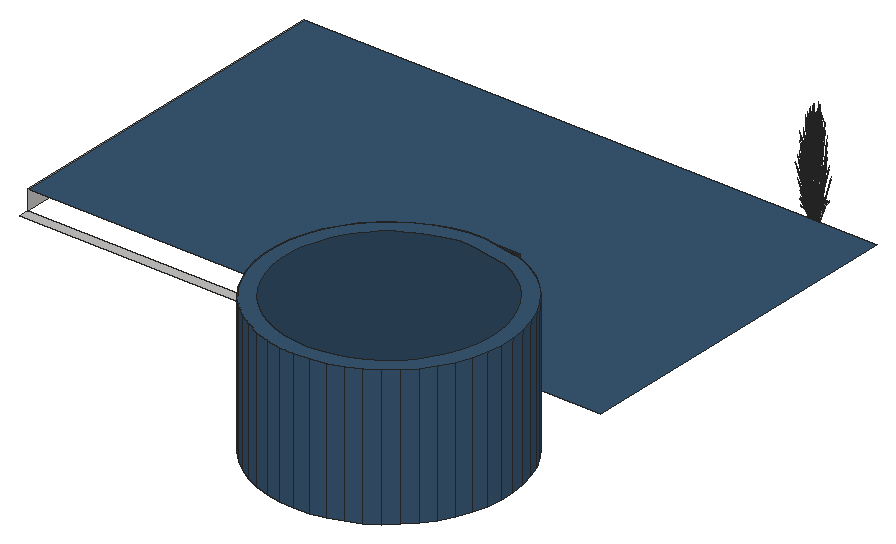
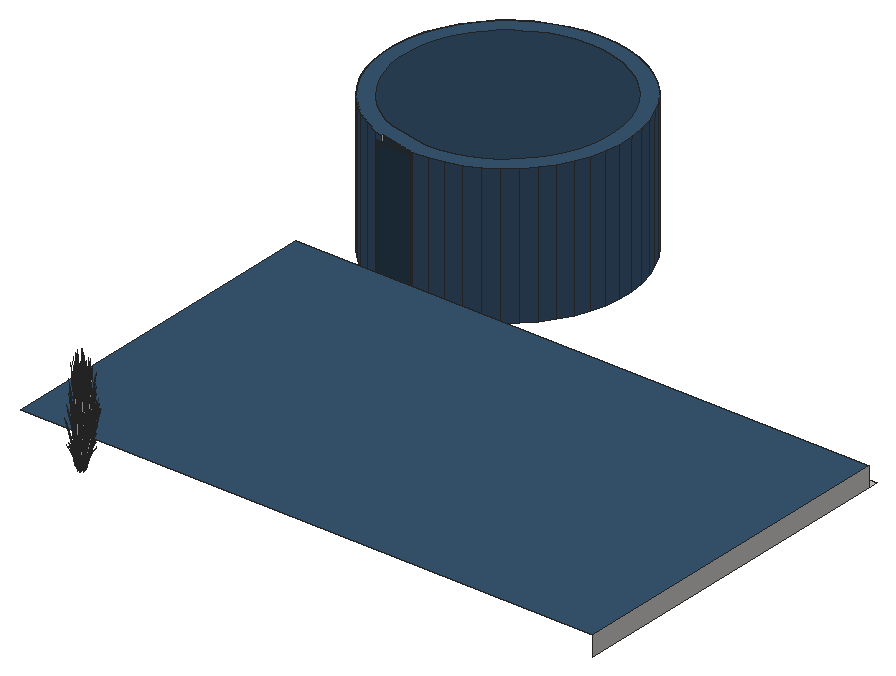
# SketchUp Ruby script. Lengths in inches.
U = 1.inch
M = Sketchup.active_model
def pt(a) = Geom::Point3d.new(a.map { |v| v * U })
def face(e, loops, mat)
  f = e.add_face(loops[0].map { |a| pt(a) })
  loops[1..].each { |l| e.add_face(l.map { |a| pt(a) }).erase! }
  f.material = f.back_material = mat if mat
  f
end
# faces: each face lists its corners as indices into pts; further lists are holes
def faces(e, pts, list, mat = nil) = list.each { |f| face(e, (f[0].is_a?(Array) ? f : [f]).map { |l| l.map { |i| pts[i] } }, mat) }
# xy, xz, yz: faces in a plane at the given z, y or x. An outline is a flat list of corners, or four numbers for a rectangle; further outlines are holes
def ring(l) = l.size == 4 ? [[l[0], l[1]], [l[2], l[1]], [l[2], l[3]], [l[0], l[3]]] : l.each_slice(2).to_a
def flat(e, list, mat, &to3) = list.each { |f| face(e, (f[0].is_a?(Array) ? f : [f]).map { |l| ring(l).map { |u, v| to3.(u, v) } }, mat) }
def xy(e, z, list, mat = nil) = flat(e, list, mat) { |x, y| [x, y, z] }
def xz(e, y, list, mat = nil) = flat(e, list, mat) { |x, z| [x, y, z] }
def yz(e, x, list, mat = nil) = flat(e, list, mat) { |y, z| [x, y, z] }
def lines(e, pts, list) = list.each { |a, b| e.add_line(pt(pts[a]), pt(pts[b])) }
# prism: a flat outline (further loops are holes) pulled along v
def prism(e, loops, v, mat = nil)
  f = face(e, loops, mat); d = Geom::Vector3d.new(v.map { |x| x * U })
  f.pushpull(f.normal.samedirection?(d) ? d.length : -d.length)
end
def box(e, o, s, mat = nil) = prism(e, [[o, [o[0] + s[0], o[1], o[2]], [o[0] + s[0], o[1] + s[1], o[2]], [o[0], o[1] + s[1], o[2]]]], [0, 0, s[2]], mat)
def at(x, y, z, deg = 0) = Geom::Transformation.translation(pt([x, y, z])) * Geom::Transformation.rotation(ORIGIN, Z_AXIS, deg.degrees)
def axes(o, x, y, z) = Geom::Transformation.new([*x, 0, *y, 0, *z, 0, *pt(o).to_a, 1])
def part(name) = M.definitions.add(name)
# library, detail: a bought-in or finely detailed component or shape, given as its bounding box
def library(name, o, s) = part(name).tap { |d| box(d.entities, o, s) }
def detail(e, o, s) = box(e.add_group.entities, o, s)
def put(e, d, t, mat = nil) = e.add_instance(d, t).tap { |i| i.material = mat if mat }
def group(e, t, mat = nil) = e.add_group.tap { |g| g.transformation = t; g.material = mat if mat }.entities
root = M.entities
M.materials.add("Carpet_01_1K").color = [196, 195, 193]
M.materials.add("Carpet_04_1K").color = [56, 85, 112]
M.materials.add("Carpet_04_1K1").color = [43, 65, 85]
M.materials.add("LightPink_Translucent").color = [144, 107, 117]
M.materials["LightPink_Translucent"].alpha = 0.75
c1 = part("blade")
p = [[2.15,0.21,22],[0,0.17,0],[0.09,0.45,0],[2.18,0.31,22],[2.29,0.31,22],[0.38,0.45,0],
  [2.48,0.24,33],[2.49,0.24,33],[2.48,0.22,33]]
faces(c1.entities,p,[[0,1,2,3],[4,5,2,3],[6,3,4,7],[8,0,3,6]])
c2 = part("seeds")
p = [[0.3,-0.1,1.38],[-0.01,-0.03,1.59],[-0.01,-0.03,0.03],[0.14,-0.07,-0.07],[0.29,-0.03,3],[0.15,0.01,3.11]]
faces(c2.entities,p,[[0,1,2,3],[1,0,4,5]],"LightPink_Translucent")
c3 = part("blade with seeds")
put(c3.entities,c1,at(0,0,0))
put(c3.entities,c2,axes([2.4,0.25,30.99],[1.5799,-0.05474,1.17369],[-0.12525,1.92788,0.29478],[-0.07173,-0.02425,1.56792]))
xy(root,1398,[[330.57,149.5,330.57,150.21,326.6875,151.48,317.8,153.17,311.55,153.5625,309.76,153.55],[330.57,150.21,330.57,153.74,311.55,153.5625,317.8,153.17,326.6875,151.48],[309.76,153.55,311.55,153.5625,308.78,153.74],[311.55,153.5625,330.57,153.74,308.78,153.74]])
xy(root,1398,[[186.57,149.5,308.78,153.74,330.57,153.74,330.57,155.5,30.57,155.5,30.57,149.51,186.57,149.51]],"Carpet_01_1K")
xy(root,1410,[[30.57,155.5,378.57,364.54]],"Carpet_04_1K")
xy(root,1482,[[[308.78,9.74,317.8,10.31,326.6875,12,335.29,14.79,343.47,18.64,351.1,23.49,358.07,29.25,364.26,35.84,369.57,43.16,373.93,51.08,377.26,59.49,379.51,68.25,380.64,77.22,380.64,86.26,379.51,95.23,377.26,103.99,373.93,112.39,369.57,120.32,364.26,127.63,358.07,134.22,351.1,139.99,343.47,144.83,335.29,148.68,330.57,150.21,330.57,149.5,308.78,153.74,299.76,153.17,290.875,151.48,282.28,148.68,274.09,144.83,266.46,139.99,259.49,134.22,253.3,127.63,247.99,120.32,243.63,112.39,240.3,103.99,238.06,95.23,236.92,86.26,236.92,77.22,238.06,68.25,240.3,59.49,243.63,51.08,247.99,43.16,253.3,35.84,259.49,29.25,266.46,23.49,274.09,18.64,282.28,14.79,290.875,12,299.76,10.31],[308.78,18.76,300.89,19.25,293.12,20.73,285.6,23.18,278.4375,26.55,271.76,30.78,265.67,35.83,260.25,41.59,255.6,47.99,251.79,54.92,248.88,62.28,246.91,69.9375,245.92,77.78,245.92,85.69,246.91,93.54,248.88,101.2,251.79,108.55,255.6,115.49,260.25,121.88,265.67,127.65,271.76,132.69,278.4375,136.93,285.6,140.3,293.12,142.74,300.89,144.22,308.19,144.68,332.82,139.9,339.12,136.93,345.8,132.69,351.89,127.65,357.31,121.88,361.96,115.49,365.77,108.55,368.68,101.2,370.65,93.54,371.64,85.69,371.64,77.78,370.65,69.9375,368.68,62.28,365.77,54.92,361.96,47.99,357.31,41.59,351.89,35.83,345.8,30.78,339.12,26.55,331.97,23.18,324.44,20.73,316.67,19.25]]],"Carpet_04_1K")
xy(root,1482,[[308.78,18.76,316.67,19.25,324.44,20.73,331.97,23.18,339.12,26.55,345.8,30.78,351.89,35.83,357.31,41.59,361.96,47.99,365.77,54.92,368.68,62.28,370.65,69.9375,371.64,77.78,371.64,85.69,370.65,93.54,368.68,101.2,365.77,108.55,361.96,115.49,357.31,121.88,351.89,127.65,345.8,132.69,339.12,136.93,332.82,139.9,308.19,144.68,300.89,144.22,293.12,142.74,285.6,140.3,278.4375,136.93,271.76,132.69,265.67,127.65,260.25,121.88,255.6,115.49,251.79,108.55,248.88,101.2,246.91,93.54,245.92,85.69,245.92,77.78,246.91,69.9375,248.88,62.28,251.79,54.92,255.6,47.99,260.25,41.59,265.67,35.83,271.76,30.78,278.4375,26.55,285.6,23.18,293.12,20.73,300.89,19.25]],"Carpet_04_1K1")
yz(root,30.57,[[155.5,1398,364.54,1410]],"Carpet_01_1K")
yz(root,236.92,[[77.22,1398,86.26,1482]],"Carpet_04_1K")
yz(root,330.57,[[149.5,1398,150.21,1482]])
yz(root,380.64,[[77.22,1398,86.26,1482]],"Carpet_04_1K")
p = [[299.76,10.31,1482],[299.76,10.31,1398],[308.78,9.74,1398],[308.78,9.74,1482],[317.8,10.31,1398],[317.8,10.31,1482],
  [290.875,12,1482],[290.875,12,1398],[326.6875,12,1398],[326.6875,12,1482],[282.28,14.79,1482],[282.28,14.79,1398],
  [335.29,14.79,1398],[335.29,14.79,1482],[274.09,18.64,1482],[274.09,18.64,1398],[343.47,18.64,1398],[343.47,18.64,1482],
  [266.46,23.49,1482],[266.46,23.49,1398],[351.1,23.49,1398],[351.1,23.49,1482],[259.49,29.25,1482],[259.49,29.25,1398],
  [358.07,29.25,1398],[358.07,29.25,1482],[253.3,35.84,1482],[253.3,35.84,1398],[364.26,35.84,1398],[364.26,35.84,1482],
  [247.99,43.16,1482],[247.99,43.16,1398],[369.57,43.16,1398],[369.57,43.16,1482],[243.63,51.08,1482],[243.63,51.08,1398],
  [373.93,51.08,1398],[373.93,51.08,1482],[240.3,59.49,1482],[240.3,59.49,1398],[377.26,59.49,1398],[377.26,59.49,1482],
  [238.06,68.25,1482],[238.06,68.25,1398],[379.51,68.25,1398],[379.51,68.25,1482],[236.92,77.22,1482],[236.92,77.22,1398],
  [380.64,77.22,1398],[380.64,77.22,1482],[238.06,95.23,1482],[238.06,95.23,1398],[236.92,86.26,1398],[236.92,86.26,1482],
  [380.64,86.26,1482],[380.64,86.26,1398],[379.51,95.23,1398],[379.51,95.23,1482],[240.3,103.99,1482],[240.3,103.99,1398],
  [377.26,103.99,1398],[377.26,103.99,1482],[243.63,112.39,1482],[243.63,112.39,1398],[373.93,112.39,1398],[373.93,112.39,1482],
  [247.99,120.32,1482],[247.99,120.32,1398],[369.57,120.32,1398],[369.57,120.32,1482],[253.3,127.63,1482],[253.3,127.63,1398],
  [364.26,127.63,1398],[364.26,127.63,1482],[259.49,134.22,1482],[259.49,134.22,1398],[358.07,134.22,1398],[358.07,134.22,1482],
  [266.46,139.99,1482],[266.46,139.99,1398],[351.1,139.99,1398],[351.1,139.99,1482],[274.09,144.83,1482],[274.09,144.83,1398],
  [343.47,144.83,1398],[343.47,144.83,1482],[282.28,148.68,1482],[282.28,148.68,1398],[335.29,148.68,1398],[335.29,148.68,1482],
  [290.875,151.48,1482],[290.875,151.48,1398],[330.57,150.21,1398],[330.57,150.21,1482],[330.57,149.5,1398],[309.76,153.55,1398],
  [309.76,153.55,1399],[329.59,149.69,1399],[329.59,149.69,1481],[309.76,153.55,1481],[308.78,153.74,1398],[308.78,153.74,1482],
  [330.57,149.5,1482],[299.76,153.17,1482],[299.76,153.17,1398],[330.57,153.74,1398],[311.55,153.5625,1398],[330.57,153.74,1481],
  [310.76,153.56,1480],[310.76,153.56,1399],[311.55,153.5625,1399],[329.58,153.73,1399],[329.58,153.73,1480]]
faces(root,p,[[0,1,2,3],[3,2,4,5],[6,7,1,0],[5,4,8,9],[10,11,7,6],[9,8,12,13],[14,15,11,10],[13,12,16,17],
  [18,19,15,14],[17,16,20,21],[22,23,19,18],[21,20,24,25],[26,27,23,22],[25,24,28,29],[30,31,27,26],[29,28,32,33],
  [34,35,31,30],[33,32,36,37],[38,39,35,34],[37,36,40,41],[42,43,39,38],[41,40,44,45],[46,47,43,42],[45,44,48,49],
  [50,51,52,53],[54,55,56,57],[58,59,51,50],[57,56,60,61],[62,63,59,58],[61,60,64,65],[66,67,63,62],[65,64,68,69],
  [70,71,67,66],[69,68,72,73],[74,75,71,70],[73,72,76,77],[78,79,75,74],[77,76,80,81],[82,83,79,78],[81,80,84,85],
  [86,87,83,82],[85,84,88,89],[90,91,87,86],[89,88,92,93],[103,104,91,90],[101,100,104,103]],"Carpet_04_1K")
faces(root,p,[[94,95,96,97,98,99,96,95,100,101,102],[[105,106,95,96,99,107],[108,109,110,111,112]],[96,99,98,97],[109,108,112,111,110]],"Carpet_04_1K1")
put(root,c3,axes([330.27,376.06,1401.875],[0.08068,0.14973,1.71376],[-0.3728,0.12606,0.13857],[-0.08426,-0.23506,0.73262]))
put(root,c3,axes([330.89,375.07,1402.72],[-0.05398,-0.06539,1.74944],[-0.36026,0.04145,-0.27667],[-0.0575,-0.15639,0.14031]))
put(root,c3,axes([331.72,375.84,1400.59],[-0.10032,0.0944,1.43002],[-0.30046,-0.16522,-0.30754],[0.05569,-0.20547,0.61141]))
put(root,c3,axes([331.27,376.17,1402.98],[-0.16845,-0.3792,-0.71045],[0.34676,-0.21133,0.08574],[-0.03939,-0.18322,1.00501]))
put(root,c3,axes([330.17,375.66,1400.59],[-0.02137,0.15256,1.43002],[-0.31245,0.12771,-0.30754],[-0.07303,-0.19719,0.61141]))
put(root,c3,axes([330.98,375.33,1399.49],[-0.0592,0.0168,1.76342],[-0.32738,-0.18913,-0.26939],[0.00549,-0.15776,0.30037]))
put(root,c3,axes([331.97,376.54,1402.98],[0.00918,-0.43138,-0.71045],[0.38672,0.02897,0.08574],[0.04081,-0.18275,1.00501]))
put(root,c3,axes([332.51,375.87,1402.72],[-0.00341,-0.09282,1.74944],[-0.28775,-0.26825,-0.27667],[0.04449,-0.16261,0.14031]))
put(root,c3,axes([331.3,375.85,1402.53],[0.1064,-0.35863,-0.35414],[0.31043,0.1046,0.4572],[-0.02846,-0.14439,0.87481]))
put(root,c3,axes([331.53,376.32,1401.875],[-0.06572,0.16029,1.71376],[-0.27569,-0.33172,0.13857],[0.12437,-0.20675,0.73262]))
put(root,c3,axes([332.43,375.53,1402.71],[-0.03584,0.03562,1.77383],[-0.35118,-0.12018,-0.16761],[-0.01271,-0.15545,0.31391]))
put(root,c3,axes([331.14,376.09,1402.68],[-0.34695,-0.11691,-0.51099],[0.11892,-0.40083,-0.3958],[-0.03181,-0.16138,0.97773]))
put(root,c3,axes([331.35,375.09,1400.77],[0.04528,0.27194,1.1486],[-0.25117,-0.15062,0.84392],[0.02703,-0.13924,0.25299]))
put(root,c3,axes([331.89,376.4,1402.68],[-0.25266,-0.31335,-0.51099],[0.2669,-0.27442,-0.3958],[0.03844,-0.15921,0.97773]))
put(root,c3,axes([330.52,374.85,1402.71],[-0.00658,0.0559,1.77383],[-0.32474,0.20287,-0.16761],[-0.09556,-0.1037,0.31391]))
put(root,c3,axes([330.45,375.84,1403.09],[0.39316,-0.11987,0.53763],[0.06823,0.47021,0.4433],[-0.09247,-0.13858,1.11249]))
put(root,c3,axes([331.34,375.93,1402.73],[0.34777,0.12192,0.48003],[-0.11892,0.40083,0.3958],[-0.0209,-0.15763,0.9933]))
put(root,c3,axes([331.4375,376.08,1403.03],[-0.34538,0.21713,-0.1216],[-0.16972,-0.38536,-0.67495],[-0.04557,-0.16239,1.02557]))
put(root,c3,axes([332.15,376.5625,1403.03],[-0.3879,-0.02311,-0.1216],[0.0106,-0.43749,-0.67495],[0.02694,-0.1685,1.02557]))
put(root,c3,axes([332.13,376.28,1402.53],[0.23881,-0.24554,-0.35414],[0.22606,0.28036,0.4572],[0.0344,-0.14245,0.87481]))
put(root,c3,axes([330.0625,375.42,1400.77],[0.18411,0.16231,1.1486],[-0.26813,0.09757,0.84392],[-0.05737,-0.12474,0.25299]))
put(root,c3,axes([331.43,375.9,1402.73],[0.26007,-0.1585,0.0643],[0.12729,0.28902,0.50621],[-0.02512,-0.1274,0.77189]))
put(root,c3,axes([330.51,376.28,1402.98],[-0.30095,-0.22541,-0.71045],[0.21388,-0.395,0.08574],[-0.10904,-0.13459,1.00501]))
put(root,c3,axes([330.4,375.98,1402.53],[-0.05451,-0.37564,-0.35414],[0.31161,-0.09919,0.4572],[-0.0837,-0.10765,0.87481]))
put(root,c3,axes([330.54,375.95,1402.73],[0.16041,-0.29625,0.0643],[0.22843,0.17248,0.50621],[-0.07385,-0.09498,0.77189]))
put(root,c3,axes([329.92,375.91,1399.49],[-0.03419,0.06144,1.76342],[-0.3455,0.13246,-0.26939],[-0.08346,-0.12049,0.30037]))
put(root,c3,axes([330.49,377.59,1400.1],[-0.14494,-0.47823,-0.69835],[0.41752,-0.17223,-0.18329],[-0.01602,-0.16194,1.54149]))
put(root,c3,axes([329.73,376.53,1401.875],[0.1311,0.08035,1.71376],[-0.27131,0.33708,0.13857],[-0.16909,-0.15206,0.73262]))
put(root,c3,axes([332.43,376.13,1399.49],[-0.05283,-0.03674,1.76342],[-0.13569,-0.41045,-0.26939],[0.09154,-0.11138,0.30037]))
put(root,c3,axes([331.33,376.23,1403.05],[-0.1064,0.35863,0.35414],[-0.31043,-0.1046,-0.4572],[-0.02846,-0.14439,0.87481]))
put(root,c3,axes([330.37,376.29,1402.68],[-0.34827,0.11086,-0.51099],[-0.06092,-0.41983,-0.3958],[-0.09354,-0.12031,0.97773]))
put(root,c3,axes([332.125,376.38,1402.73],[0.25132,0.3182,0.48003],[-0.2669,0.27442,0.3958],[0.04636,-0.14929,0.9933]))
put(root,c3,axes([330.61,375.91,1403.43],[-0.23555,0.44708,-0.13619],[-0.34112,-0.25757,-0.75594],[-0.11858,-0.12631,1.14864]))
put(root,c3,axes([332.22,376.41,1402.73],[0.29004,0.02173,0.0643],[-0.00795,0.32812,0.50621],[0.03035,-0.12569,0.77189]))
put(root,c3,axes([332,376.63,1403.05],[-0.23881,0.24554,0.35414],[-0.22606,-0.28036,-0.4572],[0.0344,-0.14245,0.87481]))
put(root,c3,axes([332.42,377.29,1402.98],[0.18436,-0.36797,-0.71045],[0.32306,0.26151,0.08574],[0.11008,-0.13332,1.00501]))
put(root,c3,axes([330.43,376.22,1400.375],[-0.22066,-0.46731,0],[0.36918,-0.26061,-0.51607],[0.08408,-0.05936,1.63711]))
put(root,c3,axes([332.41,377.12,1402.68],[-0.09067,-0.42583,-0.51099],[0.34336,-0.07449,-0.3958],[0.0984,-0.11438,0.97773]))
put(root,c3,axes([330.92,375.66,1400.13],[-0.2439,0.26754,-0.03893],[-0.22348,-0.29302,-0.17649],[-0.01573,-0.08303,0.58215]))
put(root,c3,axes([329.71,375.79,1402.72],[-0.07594,-0.00329,1.74944],[-0.24177,0.32918,-0.27667],[-0.129,-0.06726,0.14031]))
put(root,c3,axes([332.58,377.42,1403.03],[-0.32648,-0.25715,-0.1216],[0.18809,-0.3724,-0.67495],[0.09224,-0.12945,1.02557]))
put(root,c3,axes([331.23,378.83,1401.33],[0.305,0.18805,1.51261],[-0.29879,0.40513,0.59816],[-0.13384,-0.24012,1.26806]))
put(root,c3,axes([330.59,376.29,1403.05],[0.05451,0.37564,0.35414],[-0.31161,0.09919,-0.4572],[-0.0837,-0.10765,0.87481]))
put(root,c3,axes([329.63,377.53,1400.02],[0,-0.46636,-0.49651],[0.39487,0,0],[0,-0.10622,1.57504]))
put(root,c3,axes([330.73,376.15,1400.02],[0.33032,-0.23318,-0.49651],[0.19744,0.41812,0],[0.07523,-0.05311,1.57504]))
put(root,c3,axes([332.69,376.95,1400.59],[-0.12609,-0.01381,1.43002],[-0.12917,-0.37055,-0.30754],[0.1549,-0.10482,0.61141]))
put(root,c3,axes([329.65,376.53,1403.09],[0.29147,-0.34417,0.53763],[0.25138,0.3655,0.4433],[-0.13675,-0.06349,1.11249]))
put(root,c3,axes([333.38,377.3125,1402.71],[-0.0461,-0.00354,1.77383],[-0.19143,-0.37951,-0.16761],[0.07688,-0.12478,0.31391]))
put(root,c3,axes([331.12,377.1,1400.06],[0.23773,-0.35053,-0.62353],[0.29532,0.31785,-0.16365],[0.09526,-0.08744,1.37633]))
put(root,c3,axes([332.84,376.27,1400.77],[-0.11756,0.2374,1.1486],[-0.10105,-0.31895,0.84392],[0.09709,-0.07992,0.25299]))
put(root,c3,axes([332.67,377.16,1402.53],[0.30722,-0.06665,-0.35414],[0.08112,0.381,0.4572],[0.08804,-0.10234,0.87481]))
put(root,c3,axes([329.78,376.53,1402.73],[0.01777,-0.35463,0.0643],[0.26836,0.00972,0.50621],[-0.1028,-0.03711,0.77189]))
put(root,c3,axes([330.71,377.72,1400.21],[0.17124,-0.42022,-0.44739],[0.35581,0.20224,0.21531],[0,-0.09687,1.43643]))
put(root,c3,axes([329.68,376.64,1402.53],[-0.20082,-0.29199,-0.35414],[0.2293,-0.2764,0.4572],[-0.1165,-0.04206,0.87481]))
put(root,c3,axes([330.86,377.51,1400.67],[-0.04113,-0.53214,-0.29095],[0.42835,-0.03218,-0.50002],[0.07543,-0.07088,1.59708]))
put(root,c3,axes([329.8,377.54,1400.03],[0.24637,-0.29097,-0.30978],[0.24637,0.29097,0.30978],[0,-0.09372,1.38974]))
put(root,c3,axes([329.7,376.14,1400.13],[-0.10181,0.3808,-0.03893],[-0.31336,-0.11714,-0.17649],[-0.04758,-0.06228,0.58215]))
put(root,c3,axes([332.42,377.39,1403.05],[-0.30722,0.06665,0.35414],[-0.08112,-0.381,-0.4572],[0.08804,-0.10234,0.87481]))
put(root,c3,axes([330.67,378.07,1400.67],[-0.39748,-0.22252,-0.29095],[0.19139,-0.46966,-0.50002],[-0.01249,-0.11531,1.59708]))
put(root,c3,axes([329.53,377.88,1400.375],[-0.44133,0,0],[0,-0.52122,-0.51607],[0,-0.11871,1.63711]))
put(root,c3,axes([329.61,376.95,1400.59],[0.06891,0.12984,1.43002],[-0.15879,0.35293,-0.30754],[-0.16304,-0.08436,0.61141]))
put(root,c3,axes([330.81,376.33,1400.03],[0.32928,0.11539,-0.30978],[-0.08291,0.40636,0.30978],[0.06638,-0.04686,1.38974]))
put(root,c3,axes([329.89,376.84,1402.98],[-0.35281,-0.01123,-0.71045],[0.0237,-0.47284,0.08574],[-0.14947,-0.0499,1.00501]))
put(root,c3,axes([332.7,377.33,1402.73],[0.2423,0.19613,0.0643],[-0.14107,0.2793,0.50621],[0.07768,-0.0903,0.77189]))
put(root,c3,axes([332.63,377.25,1402.73],[0.08753,0.42921,0.48003],[-0.34336,0.07449,0.3958],[0.1012,-0.10094,0.9933]))
put(root,c3,axes([333.55,377.77,1402.72],[0.04898,-0.07104,1.74944],[-0.06269,-0.43574,-0.27667],[0.12289,-0.08262,0.14031]))
put(root,c3,axes([329.875,377.74,1400.33],[-0.32829,0.39208,0.30756],[-0.32849,-0.38796,-0.36492],[-0.01146,-0.11134,1.64885]))
put(root,c3,axes([329.42,376.07,1402.71],[0.02617,0.04654,1.77383],[-0.12614,0.41836,-0.16761],[-0.12775,0.00303,0.31391]))
put(root,c3,axes([330.92,377.93,1400.43],[0.39767,0.22603,0.24065],[-0.19139,0.46966,0.50002],[0,-0.10827,1.60543]))
put(root,c3,axes([330.77,378.5625,1400.4375],[0.09355,-0.55261,-0.23429],[0.44354,0.09633,0.51271],[-0.0775,-0.07631,1.5644]))
put(root,c3,axes([329.78,376.93,1402.68],[-0.25628,0.30892,-0.51099],[-0.22444,-0.32634,-0.3958],[-0.13021,-0.047,0.97773]))
put(root,c3,axes([329.97,376.79,1403.05],[0.20082,0.29199,0.35414],[-0.2293,0.2764,-0.4572],[-0.1165,-0.04206,0.87481]))
put(root,c3,axes([329.2,377.34,1400.77],[0.22533,-0.03337,1.1486],[-0.14293,0.29403,0.84392],[-0.11135,-0.04411,0.25299]))
put(root,c3,axes([330.79,377.61,1400.72],[-0.38326,0.02879,0.44739],[-0.03466,-0.47788,-0.21531],[0.06861,-0.04843,1.43643]))
put(root,c3,axes([329.91,376.61,1403.03],[-0.0189,0.47427,-0.1216],[-0.35781,-0.01296,-0.67495],[-0.13781,-0.03295,1.02557]))
put(root,c3,axes([329.8,377.96,1400.48],[0,0.46636,0.49651],[-0.39487,0,0],[0,-0.10622,1.57504]))
put(root,c3,axes([332.59,378.43,1403.03],[-0.17758,-0.42229,-0.1216],[0.31518,-0.20752,-0.67495],[0.13282,-0.05572,1.02557]))
put(root,c3,axes([332.57,378.06,1402.68],[0.09562,-0.42421,-0.51099],[0.32782,0.1454,-0.3958],[0.13199,-0.0389,0.97773]))
put(root,c3,axes([332.06,376.34,1400.375],[0.22066,-0.46731,0],[0.36918,0.26061,-0.51607],[0.08408,0.05936,1.63711]))
put(root,c3,axes([329.46,377.26,1401.875],[0.14639,-0.01056,1.71376],[-0.09712,0.45778,0.13857],[-0.20862,-0.02831,0.73262]))
put(root,c3,axes([330.73,378.34,1400.21],[-0.21202,-0.39143,-0.44739],[0.32115,-0.27564,0.21531],[-0.06861,-0.04843,1.43643]))
put(root,c3,axes([330.78,377.78,1400.36],[0.15345,0.52148,0.45755],[-0.43845,0.18134,0.17955],[0.00536,-0.09582,1.58856]))
put(root,c3,axes([332.92,378.18,1399.98],[-0.22732,0.05597,1.41583],[-0.03618,-0.44548,0.08104],[0.15921,-0.06743,0.80566]))
put(root,c3,axes([333.34,377.79,1400.26],[-0.21881,-0.29821,-0.06488],[0.23965,-0.27324,-0.29416],[0.0679,-0.01924,0.97024]))
put(root,c3,axes([330.7,378.2,1400.72],[-0.17124,0.42022,0.44739],[-0.35581,-0.20224,-0.21531],[0,-0.09687,1.43643]))
put(root,c3,axes([331.33,377.83,1400.21],[0,-0.53961,0],[0.44133,0,0],[0,0,1.79456]))
put(root,c3,axes([331.87,376.58,1400.48],[-0.33032,-0.23318,0.49651],[0.19744,-0.41812,0],[0.07523,0.05311,1.57504]))
put(root,c3,axes([332.51,378.22,1402.98],[0.31014,-0.20596,-0.71045],[0.17284,0.42397,0.08574],[0.14985,-0.04816,1.00501]))
put(root,c3,axes([330.54,378.49,1400.06],[-0.36714,-0.07646,-0.62353],[0.07747,-0.47163,-0.16365],[-0.10956,-0.05715,1.37633]))
put(root,c3,axes([331.12,377.49,1400.36],[-0.29264,0.42323,0.45755],[-0.34767,-0.3736,0.17955],[0.07055,-0.04224,1.58856]))
put(root,c3,axes([331.44,378.25,1400.3],[-0.32829,-0.4014,-0.06131],[0.32849,-0.40164,0],[-0.01146,-0.01402,1.75571]))
put(root,c3,axes([330.61,376.79,1400.47],[-0.10196,0.46348,0.17642],[-0.3731,-0.13116,0.35086],[0.06445,-0.00226,1.60407]))
put(root,c3,axes([332.47,378.3,1403.05],[-0.29332,-0.1301,0.35414],[0.08555,-0.37955,-0.4572],[0.11809,-0.0348,0.87481]))
put(root,c3,axes([329.4,377.61,1402.73],[0.09971,-0.42522,0.48003],[0.32782,0.1454,0.3958],[-0.12892,0.02555,0.9933]))
put(root,c3,axes([330.46,377.17,1399.59],[-0.3474,0.18671,1.28929],[-0.11057,-0.53572,0.50096],[0.21332,0.00891,1.46642]))
put(root,c3,axes([331.39,377.31,1400.62],[0.06809,-0.4162,0.1448],[0.33266,0.07225,-0.41347],[0.06054,0.04274,1.26744]))
put(root,c3,axes([329.37,377.49,1402.73],[-0.12963,-0.31798,0.0643],[0.23638,-0.15564,0.50621],[-0.1042,0.03071,0.77189]))
put(root,c3,axes([330.82,378.3,1400.36],[0.44609,0.09826,0.45755],[-0.09078,0.55493,0.17955],[-0.06519,-0.05359,1.58856]))
put(root,c3,axes([333.17,377.89,1399.49],[-0.01845,-0.0708,1.76342],[0.12793,-0.41416,-0.26939],[0.12905,-0.00596,0.30037]))
put(root,c3,axes([329.36,377.82,1399.49],[0.00895,0.0735,1.76342],[-0.18044,0.38382,-0.26939],[-0.12817,-0.01935,0.30037]))
put(root,c3,axes([331.25,377.42,1400.72],[-0.21202,-0.39143,0.44739],[0.32115,-0.27564,-0.21531],[0.06861,0.04843,1.43643]))
put(root,c3,axes([330.15,379.21,1400.03],[-0.08291,-0.40636,-0.30978],[0.32928,-0.11539,0.30978],[-0.06638,-0.04686,1.38974]))
put(root,c3,axes([330.58,379.18,1400.47],[0.37926,-0.12378,0.17642],[0.09365,0.46065,0.35086],[-0.03382,-0.06712,1.60407]))
put(root,c3,axes([331.36,377.44,1400.67],[0.35635,-0.30962,-0.29095],[0.23697,0.43749,-0.50002],[0.08792,0.04443,1.59708]))
put(root,c3,axes([332.78,378.26,1402.53],[0.29332,0.1301,-0.35414],[-0.08555,0.37955,0.4572],[0.11809,-0.0348,0.87481]))
put(root,c3,axes([330.0625,379.38,1400.02],[-0.33032,-0.23318,-0.49651],[0.19744,-0.41812,0],[-0.07523,-0.05311,1.57504]))
put(root,c3,axes([332.26,376.62,1400.02],[0.33032,0.23318,-0.49651],[-0.19744,0.41812,0],[0.07523,0.05311,1.57504]))
put(root,c3,axes([329.33,377.65,1402.53],[-0.29332,-0.1301,-0.35414],[0.08555,-0.37955,0.4572],[-0.11809,0.0348,0.87481]))
put(root,c3,axes([331.63,377.95,1400.21],[0.39487,0,0],[0,0.48281,0],[0,0,1.78407]))
put(root,c3,axes([330.96,378.56,1400.67],[-0.35635,0.30962,-0.29095],[-0.23697,-0.43749,-0.50002],[-0.08792,-0.04443,1.59708]))
put(root,c3,axes([331.74,376.82,1400.47],[-0.37926,0.12378,0.17642],[-0.09365,-0.46065,0.35086],[0.03382,0.06712,1.60407]))
put(root,c3,axes([331.98,377.79,1401.875],[-0.14639,0.01056,1.71376],[0.09712,-0.45778,0.13857],[0.20862,0.02831,0.73262]))
put(root,c3,axes([332.17,376.79,1400.03],[0.08291,0.40636,-0.30978],[-0.32928,0.11539,0.30978],[0.06638,0.04686,1.38974]))
put(root,c3,axes([332.73,378.42,1402.73],[0.12963,0.31798,0.0643],[-0.23638,0.15564,0.50621],[0.1042,-0.03071,0.77189]))
put(root,c3,axes([331.5,377.7,1400.38],[-0.44609,-0.09826,0.49198],[0.09078,-0.55493,0.19306],[0.06519,0.05359,1.70813]))
put(root,c3,axes([332.71,378.31,1402.73],[-0.09971,0.42522,0.48003],[-0.32782,-0.1454,0.3958],[0.12892,-0.02555,0.9933]))
put(root,c3,axes([331.15,379.07,1400.2],[-0.11516,-0.40207,0],[0.32884,-0.1408,0],[0,0,1.54371]))
put(root,c3,axes([330.93,378.69,1400.62],[-0.06809,0.4162,0.1448],[-0.33266,-0.07225,-0.41347],[-0.06054,-0.04274,1.26744]))
put(root,c3,axes([329.64,377.61,1403.05],[0.29332,0.1301,0.35414],[-0.08555,0.37955,-0.4572],[-0.11809,0.0348,0.87481]))
put(root,c3,axes([331.58,379.02,1400.18],[0.37054,-0.15823,-0.19198],[0.1302,0.45581,0.00008],[0.0409,-0.01749,1.73897]))
put(root,c3,axes([331.71,379.21,1400.47],[0.10196,-0.46348,0.17642],[0.3731,0.13116,0.35086],[-0.06445,0.00226,1.60407]))
put(root,c3,axes([331.62,378.16,1400.21],[0.24637,0.30123,0],[-0.24637,0.30123,0],[0,0,1.69266]))
put(root,c3,axes([330.22,377.59,1401.34],[0.10032,-0.06746,1.77064],[0.0346,0.47103,0.13857],[-0.2173,0.0625,0.63284]))
put(root,c3,axes([332.29,378.02,1400.47],[-0.2773,-0.3397,0.17642],[0.27945,-0.32949,0.35086],[-0.03063,0.06937,1.60407]))
put(root,c3,axes([331.78,377.51,1400.06],[0.36714,0.07646,-0.62353],[-0.07747,0.47163,-0.16365],[0.10956,0.05715,1.37633]))
put(root,c3,axes([333.4,378.34,1400.77],[-0.21807,0.07699,1.1486],[0.10265,-0.31819,0.84392],[0.11568,0.02177,0.25299]))
put(root,c3,axes([331.07,379.26,1400.2],[-0.35581,-0.20937,0],[0.17124,-0.43505,0],[0,0,1.62707]))
put(root,c3,axes([331.36,378.7,1400.46],[-0.34464,-0.37536,-0.25192],[0.29,-0.42149,0.5513],[-0.0928,0.04391,1.68216]))
put(root,c3,axes([330.45,379.42,1400.48],[0.33032,0.23318,0.49651],[-0.19744,0.41812,0],[-0.07523,-0.05311,1.57504]))
put(root,c3,axes([331.62,377.8,1400.72],[0.17124,-0.42022,0.44739],[0.35581,0.20224,-0.21531],[0,0.09687,1.43643]))
put(root,c3,axes([333.3,379.68,1402.71],[-0.03191,-0.04083,1.77383],[0.06981,-0.43764,-0.16761],[0.12571,-0.02796,0.31391]))
put(root,c3,axes([329.14,377.91,1402.72],[-0.05763,0.06055,1.74944],[0.0049,0.44239,-0.27667],[-0.13211,0.05753,0.14031]))
put(root,c3,axes([331.55,378.04,1400.29],[0,0.53934,-0.05637],[-0.44133,0,0],[0,0.01695,1.79368]))
put(root,c3,axes([329.53,377.85,1402.68],[-0.09562,0.42421,-0.51099],[-0.32782,-0.1454,-0.3958],[-0.13199,0.0389,0.97773]))
put(root,c3,axes([329.51,377.48,1403.03],[0.17758,0.42229,-0.1216],[-0.31518,0.20752,-0.67495],[-0.13282,0.05572,1.02557]))
put(root,c3,axes([331.58,377.66,1400.21],[0.21202,0.39143,-0.44739],[-0.32115,0.27564,0.21531],[0.06861,0.04843,1.43643]))
put(root,c3,axes([333.02,379.32,1401.93],[-0.06755,-0.39203,-0.03492],[0.31928,-0.09013,-0.15832],[0.06667,0.02485,0.52218]))
put(root,c3,axes([330.26,379.66,1400.375],[-0.22066,0.46731,0],[-0.36918,-0.26061,-0.51607],[-0.08408,-0.05936,1.63711]))
put(root,c3,axes([332.19,379.3,1403.03],[0.0189,-0.47427,-0.1216],[0.35781,0.01296,-0.67495],[0.13781,0.03295,1.02557]))
put(root,c3,axes([332.52,378.04,1400.48],[0,-0.46636,0.49651],[0.39487,0,0],[0,0.10622,1.57504]))
put(root,c3,axes([331.53,378.39,1400.72],[0.38326,-0.02879,0.44739],[0.03466,0.47788,-0.21531],[-0.06861,0.04843,1.43643]))
put(root,c3,axes([331.77,377.9,1400.62],[0.32884,-0.136,0.1448],[0.11516,0.38837,-0.41347],[0,0.08547,1.26744]))
put(root,c3,axes([332.14,379.12,1403.05],[-0.20082,-0.29199,0.35414],[0.2293,-0.2764,-0.4572],[0.1165,0.04206,0.87481]))
put(root,c3,axes([331.1875,378.62,1400.21],[-0.38326,0.02879,-0.44739],[-0.03466,-0.47788,0.21531],[-0.06861,0.04843,1.43643]))
put(root,c3,axes([332.99,378.85,1400.59],[-0.085,-0.1147,1.43002],[0.1106,-0.37943,-0.30754],[0.17198,0.0514,0.61141]))
put(root,c3,axes([331.47,379.26,1400.2],[0.35581,0.20937,0],[-0.17124,0.43505,0],[0,0,1.74954]))
put(root,c3,axes([332.5,379.02,1402.72],[0.07571,-0.00789,1.74944],[0.20767,-0.36231,-0.27667],[0.13467,0.04783,0.14031]))
put(root,c3,axes([331.61,379.73,1400.19],[-0.21791,-0.46895,-0.05142],[0.36918,-0.26061,0.51607],[-0.09097,0.04465,1.6363]))
